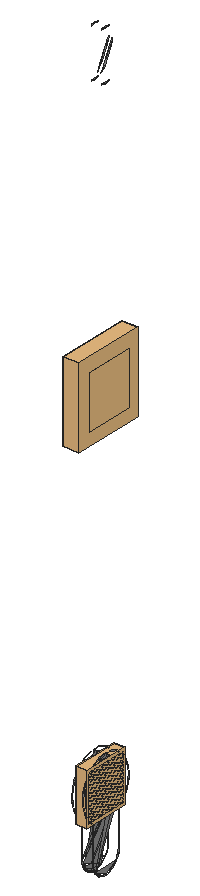
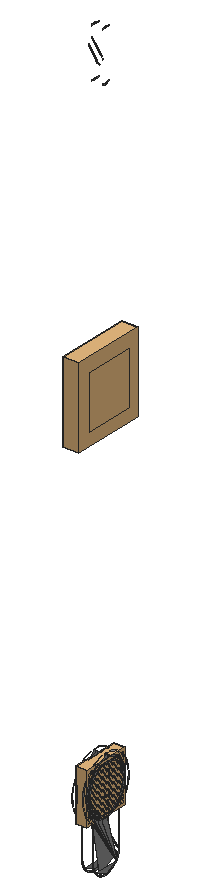
# SketchUp Ruby script. Lengths in inches.
U = 1.inch
M = Sketchup.active_model
def pt(a) = Geom::Point3d.new(a.map { |v| v * U })
def face(e, loops, mat)
  f = e.add_face(loops[0].map { |a| pt(a) })
  loops[1..].each { |l| e.add_face(l.map { |a| pt(a) }).erase! }
  f.material = f.back_material = mat if mat
  f
end
# faces: each face lists its corners as indices into pts; further lists are holes
def faces(e, pts, list, mat = nil) = list.each { |f| face(e, (f[0].is_a?(Array) ? f : [f]).map { |l| l.map { |i| pts[i] } }, mat) }
# xy, xz, yz: faces in a plane at the given z, y or x. An outline is a flat list of corners, or four numbers for a rectangle; further outlines are holes
def ring(l) = l.size == 4 ? [[l[0], l[1]], [l[2], l[1]], [l[2], l[3]], [l[0], l[3]]] : l.each_slice(2).to_a
def flat(e, list, mat, &to3) = list.each { |f| face(e, (f[0].is_a?(Array) ? f : [f]).map { |l| ring(l).map { |u, v| to3.(u, v) } }, mat) }
def xy(e, z, list, mat = nil) = flat(e, list, mat) { |x, y| [x, y, z] }
def xz(e, y, list, mat = nil) = flat(e, list, mat) { |x, z| [x, y, z] }
def yz(e, x, list, mat = nil) = flat(e, list, mat) { |y, z| [x, y, z] }
def lines(e, pts, list) = list.each { |a, b| e.add_line(pt(pts[a]), pt(pts[b])) }
# prism: a flat outline (further loops are holes) pulled along v
def prism(e, loops, v, mat = nil)
  f = face(e, loops, mat); d = Geom::Vector3d.new(v.map { |x| x * U })
  f.pushpull(f.normal.samedirection?(d) ? d.length : -d.length)
end
def box(e, o, s, mat = nil) = prism(e, [[o, [o[0] + s[0], o[1], o[2]], [o[0] + s[0], o[1] + s[1], o[2]], [o[0], o[1] + s[1], o[2]]]], [0, 0, s[2]], mat)
def at(x, y, z, deg = 0) = Geom::Transformation.translation(pt([x, y, z])) * Geom::Transformation.rotation(ORIGIN, Z_AXIS, deg.degrees)
def axes(o, x, y, z) = Geom::Transformation.new([*x, 0, *y, 0, *z, 0, *pt(o).to_a, 1])
def part(name) = M.definitions.add(name)
# library, detail: a bought-in or finely detailed component or shape, given as its bounding box
def library(name, o, s) = part(name).tap { |d| box(d.entities, o, s) }
def detail(e, o, s) = box(e.add_group.entities, o, s)
def put(e, d, t, mat = nil) = e.add_instance(d, t).tap { |i| i.material = mat if mat }
def group(e, t, mat = nil) = e.add_group.tap { |g| g.transformation = t; g.material = mat if mat }.entities
root = M.entities
M.materials.add("Material \#1").color = [140, 140, 140]
c1 = library("3DGeom~1_Defintion",[-60.87,347.29,-704.08],[121.74,121.75,1000])
c2 = library("3DGeom~13_Defintion",[-84.91,-744.98,-830.03],[169.82,169.83,1000])
c3 = library("3DGeom~14_Defintion",[-102.17,352.37,-727.27],[204.35,204.35,1000])
c4 = part("3DGeom~10_Defintion")
yz(c4.entities,-68.96,[[-797.08,-844.83,-797.08,-827.59,-922.41,-827.59],[-922.41,-844.83,-797.08,-844.83,-922.41,-827.59]],"Material \#1")
yz(c4.entities,68.97,[[-922.41,-844.83,-797.08,-827.59,-797.08,-844.83],[-922.41,-844.83,-922.41,-827.59,-797.08,-827.59],[-797.08,137.93,-922.41,155.17,-797.08,155.17],[-922.41,137.93,-922.41,155.17,-797.08,137.93]],"Material \#1")
p = [[-15.8,-989.55,-844.83],[-15.8,-989.55,-827.59],[0,-991.38,-827.59],[0,-991.38,-844.83],[15.8,-989.55,-827.59],[15.8,-989.55,-844.83],
  [-30.32,-984.36,-844.83],[-30.32,-984.36,-827.59],[30.31,-984.36,-827.59],[30.31,-984.36,-844.83],[-43.12,-976.21,-844.83],[-43.12,-976.21,-827.59],
  [43.12,-976.21,-827.59],[43.12,-976.21,-844.83],[-53.81,-965.53,-844.83],[-53.81,-965.53,-827.59],[53.8,-965.53,-827.59],[53.8,-965.53,-844.83],
  [-61.95,-952.73,-844.83],[-61.95,-952.73,-827.59],[53.8,-965.53,-827.59],[61.95,-952.73,-827.59],[61.95,-952.73,-844.83],[-67.15,-938.21,-844.83],
  [-67.15,-938.21,-827.59],[67.14,-938.21,-827.59],[67.14,-938.21,-844.83],[-68.96,-922.41,-844.83],[-68.96,-922.41,-827.59],[67.14,-938.21,-827.59],
  [68.97,-922.41,-827.59],[68.97,-922.41,-844.83],[-69.1,-794.86,-844.83],[-69.1,-794.86,-827.59],[-68.96,-797.08,-827.59],[-68.96,-797.08,-844.83],
  [68.97,-797.08,-844.83],[68.97,-797.08,-827.59],[69.11,-794.71,-827.59],[69.11,-794.71,-844.83],[-69.48,-792.73,-844.83],[-69.48,-792.73,-827.59],
  [69.53,-792.51,-827.59],[69.53,-792.51,-844.83],[-70.14,-790.6875,-844.83],[-70.14,-790.6875,-827.59],[70.24,-790.48,-827.59],[70.24,-790.48,-844.83],
  [-71.08,-788.73,-844.83],[-71.08,-788.73,-827.59],[71.22,-788.57,-827.59],[71.22,-788.57,-844.83],[-72.32,-786.86,-844.83],[-72.32,-786.86,-827.59],
  [72.47,-786.78,-827.59],[72.47,-786.78,-844.83],[-73.8,-785.17,-844.83],[-73.8,-785.17,-827.59],[74,-785.04,-827.59],[74,-785.04,-844.83],
  [-75.96,-783.21,-844.83],[-75.96,-783.21,-827.59],[74,-785.04,-827.59],[75.76,-783.39,-827.59],[75.76,-783.39,-844.83],[86.625,-772.95,-827.59],
  [86.61,-772.96,-844.83],[-86.89,-773.25,-844.83],[-86.89,-773.25,-827.59],[-75.96,-783.21,-844.83],[-96.66,-761.8,-844.83],[-96.66,-761.8,-827.59],
  [86.625,-772.95,-827.59],[86.63,-772.94,-844.83],[86.61,-772.96,-844.83],[86.625,-772.95,-827.59],[86.62,-772.95,-827.59],[86.62,-772.95,-827.59],
  [96.31,-761.375,-827.59],[96.31,-761.375,-844.83],[86.63,-772.94,-844.83],[86.625,-772.95,-827.59],[86.62,-772.95,-827.59],[-104.96,-749.18,-844.83],
  [-104.96,-749.18,-827.59],[-96.66,-761.8,-827.59],[-96.66,-761.8,-844.83],[96.31,-761.375,-827.59],[104.62,-748.77,-827.59],[104.62,-748.77,-844.83],
  [-111.64,-735.52,-844.83],[-111.64,-735.52,-827.59],[111.39,-735.21,-827.59],[111.39,-735.21,-844.83],[-116.49,-721.23,-844.83],[-116.49,-721.23,-827.59],
  [116.4375,-720.78,-827.59],[116.4375,-720.78,-844.83],[-119.64,-705.62,-844.83],[-119.64,-705.62,-827.59],[119.6,-705.57,-827.59],[119.6,-705.57,-844.83],
  [-120.6875,-689.65,-844.83],[-120.6875,-689.65,-827.59],[120.69,-689.65,-827.59],[120.69,-689.65,-844.83],[-117.5,-662,-844.83],[-117.5,-662,-827.59],
  [117.5,-662,-827.59],[117.5,-662,-844.83],[-108.41,-636.61,-844.83],[-108.41,-636.61,-827.59],[117.5,-662,-844.83],[108.41,-636.61,-827.59],
  [108.41,-636.61,-844.83],[-93.91,-613.95,-844.83],[-93.91,-613.95,-827.59],[-108.41,-636.61,-827.59],[108.41,-636.61,-844.83],[94.16,-614.19,-827.59],
  [94.16,-614.19,-844.83],[94.16,-614.19,-827.59],[75.46,-595.5,-827.59],[75.46,-595.5,-844.83],[-75.46,-595.5,-844.83],[-75.46,-595.5,-827.59],
  [-93.91,-613.95,-827.59],[-93.91,-613.95,-827.59],[-93.91,-613.95,-844.83],[-53.05,-581.24,-844.83],[-53.05,-581.24,-827.59],[-75.46,-595.5,-827.59],
  [-75.46,-595.5,-844.83],[53.05,-581.24,-827.59],[53.05,-581.24,-844.83],[-27.65,-572.16,-844.83],[-27.65,-572.16,-827.59],[-53.05,-581.24,-827.59],
  [-53.05,-581.24,-844.83],[27.66,-572.16,-827.59],[27.66,-572.16,-844.83],[0,-568.97,-844.83],[0,-568.97,-827.59],[-27.65,-572.16,-827.59],
  [-27.65,-572.16,-844.83],[0,-568.97,-844.83],[-15.8,-989.55,155.17],[0,-991.38,155.17],[0,-991.38,137.93],[-15.8,-989.55,137.93],
  [15.8,-989.55,155.17],[15.8,-989.55,137.93],[-30.32,-984.36,155.17],[-30.32,-984.36,137.93],[30.31,-984.36,155.17],[30.31,-984.36,137.93],
  [-43.125,-976.22,155.17],[-43.125,-976.22,137.93],[43.12,-976.22,155.17],[43.12,-976.22,137.93],[-53.81,-965.53,155.17],[-53.81,-965.53,137.93],
  [53.8,-965.53,155.17],[53.8,-965.53,137.93],[-61.96,-952.73,155.17],[-61.95,-952.73,137.93],[61.95,-952.73,155.17],[61.95,-952.73,137.93],
  [53.8,-965.53,137.93],[-67.15,-938.21,155.17],[-67.15,-938.21,137.93],[67.14,-938.21,155.17],[67.14,-938.21,137.93],[-68.96,-922.41,155.17],
  [-68.96,-922.41,137.93],[68.97,-922.41,155.17],[68.97,-922.41,137.93],[67.14,-938.21,137.93],[-68.97,-797.08,155.17],[-68.97,-797.08,137.93],
  [-69.1,-794.86,155.17],[-69.1,-794.86,137.93],[68.97,-797.08,155.17],[69.11,-794.71,155.17],[69.11,-794.71,137.93],[68.97,-797.08,137.93],
  [-69.48,-792.73,155.17],[-69.48,-792.73,137.93],[69.53,-792.51,155.17],[69.53,-792.51,137.93],[-70.14,-790.6875,155.17],[-70.14,-790.6875,137.93],
  [70.24,-790.48,155.17],[70.24,-790.48,137.93],[-71.08,-788.73,155.17],[-71.08,-788.73,137.93],[71.22,-788.57,155.17],[71.22,-788.57,137.93],
  [-72.32,-786.86,155.17],[-72.32,-786.86,137.93],[72.47,-786.78,155.17],[72.47,-786.78,137.93],[-73.8,-785.17,155.17],[-73.8,-785.17,137.93],
  [74,-785.04,155.17],[74,-785.04,137.93],[-75.96,-783.21,155.17],[-75.96,-783.21,137.93],[75.76,-783.39,155.17],[75.76,-783.39,137.93],
  [74,-785.04,137.93],[86.61,-772.96,155.17],[86.625,-772.95,137.93],[-86.88,-773.25,155.17],[-75.96,-783.21,155.17],[-86.88,-773.25,137.93],
  [-96.66,-761.8,155.17],[-96.66,-761.8,137.93],[86.63,-772.94,155.17],[86.625,-772.95,137.93],[86.61,-772.96,155.17],[86.62,-772.95,137.93],
  [86.625,-772.95,137.93],[96.31,-761.375,155.17],[96.31,-761.375,137.93],[86.62,-772.95,137.93],[86.63,-772.94,155.17],[86.62,-772.95,137.93],
  [86.625,-772.95,137.93],[-104.96,-749.18,155.17],[-96.66,-761.8,155.17],[-96.66,-761.8,137.93],[-104.96,-749.18,137.93],[104.62,-748.77,155.17],
  [104.62,-748.77,137.93],[96.31,-761.375,137.93],[-111.64,-735.52,155.17],[-111.64,-735.52,137.93],[111.39,-735.21,155.17],[111.39,-735.21,137.93],
  [-116.49,-721.23,155.17],[-116.49,-721.23,137.93],[116.4375,-720.78,155.17],[116.4375,-720.78,137.93],[-119.64,-705.62,155.17],[-119.64,-705.62,137.93],
  [119.6,-705.57,155.17],[119.6,-705.57,137.93],[-120.6875,-689.65,155.17],[-120.6875,-689.65,137.93],[120.69,-689.65,155.17],[120.69,-689.65,137.93],
  [-117.5,-662,155.17],[-117.5,-662,137.93],[117.5,-662,155.17],[117.5,-662,137.93],[-108.41,-636.61,155.17],[-108.41,-636.61,137.93],
  [117.5,-662,155.17],[108.41,-636.61,155.17],[108.41,-636.61,137.93],[-93.91,-613.95,155.17],[-108.41,-636.61,137.93],[-93.91,-613.95,137.93],
  [108.41,-636.61,155.17],[94.16,-614.19,155.17],[94.16,-614.19,137.93],[75.46,-595.5,155.17],[75.46,-595.5,137.93],[94.16,-614.19,137.93],
  [-75.46,-595.5,155.17],[-93.91,-613.95,155.17],[-93.91,-613.95,137.93],[-75.46,-595.5,137.93],[-53.05,-581.24,155.17],[-75.46,-595.5,155.17],
  [-75.46,-595.5,137.93],[-53.05,-581.24,137.93],[53.05,-581.24,155.17],[53.05,-581.24,137.93],[-27.65,-572.16,155.17],[-53.05,-581.24,155.17],
  [-53.05,-581.24,137.93],[-27.65,-572.16,137.93],[27.65,-572.16,155.17],[27.65,-572.16,137.93],[0,-568.97,155.17],[-27.65,-572.16,155.17],
  [-27.65,-572.16,137.93],[0,-568.97,137.93],[0,-568.97,155.17]]
faces(c4.entities,p,[[0,1,2],[2,3,0],[3,2,4],[4,5,3],[6,7,1],[1,0,6],[5,4,8],[8,9,5],
  [10,11,7],[7,6,10],[9,8,12],[12,13,9],[14,15,11],[11,10,14],[13,12,16],[16,17,13],
  [18,19,15],[15,14,18],[17,20,21],[21,22,17],[23,24,19],[19,18,23],[22,21,25],[25,26,22],
  [27,28,24],[24,23,27],[26,29,30],[30,31,26],[32,33,34],[34,35,32],[36,37,38],[38,39,36],
  [40,41,33],[33,32,40],[39,38,42],[42,43,39],[44,45,41],[41,40,44],[43,42,46],[46,47,43],
  [48,49,45],[45,44,48],[47,46,50],[50,51,47],[52,53,49],[49,48,52],[51,50,54],[54,55,51],
  [56,57,53],[53,52,56],[55,54,58],[58,59,55],[60,61,57],[57,56,60],[59,62,63],[63,64,59],
  [64,63,65],[65,66,64],[67,68,61],[61,69,67],[70,71,68],[68,67,70],[72,73,66],[74,75,76],
  [73,77,78],[78,79,73],[80,81,82],[83,84,85],[85,86,83],[79,87,88],[88,89,79],[90,91,84],
  [84,83,90],[89,88,92],[92,93,89],[94,95,91],[91,90,94],[93,92,96],[96,97,93],[98,99,95],
  [95,94,98],[97,96,100],[100,101,97],[102,103,99],[99,98,102],[101,100,104],[104,105,101],[106,107,103],
  [103,102,106],[105,104,108],[108,109,105],[110,111,107],[107,106,110],[112,108,113],[113,114,112],[115,116,117],
  [117,110,115],[118,113,119],[119,120,118],[120,121,122],[122,123,120],[124,125,126],[127,128,124],[129,130,131],
  [131,132,129],[123,122,133],[133,134,123],[135,136,137],[137,138,135],[134,133,139],[139,140,134],[141,142,143],
  [143,144,141],[140,139,142],[142,145,140],[146,147,148],[148,149,146],[147,150,151],[151,148,147],[152,146,149],
  [149,153,152],[150,154,155],[155,151,150],[156,152,153],[153,157,156],[154,158,159],[159,155,154],[160,156,157],
  [157,161,160],[158,162,163],[163,159,158],[164,160,161],[161,165,164],[162,166,167],[167,168,162],[169,164,165],
  [165,170,169],[166,171,172],[172,167,166],[173,169,170],[170,174,173],[171,175,176],[176,177,171],[178,173,174],
  [174,179,178],[180,178,179],[179,181,180],[182,183,184],[184,185,182],[186,180,181],[181,187,186],[183,188,189],
  [189,184,183],[190,186,187],[187,191,190],[188,192,193],[193,189,188],[194,190,191],[191,195,194],[192,196,197],
  [197,193,192],[198,194,195],[195,199,198],[196,200,201],[201,197,196],[202,198,199],[199,203,202],[200,204,205],
  [205,201,200],[206,202,203],[203,207,206],[204,208,209],[209,210,204],[208,211,212],[212,209,208],[213,214,207],
  [207,215,213],[216,213,215],[215,217,216],[211,218,219],[220,221,222],[218,223,224],[224,225,218],[226,227,228],
  [229,230,231],[231,232,229],[223,233,234],[234,235,223],[236,229,232],[232,237,236],[233,238,239],[239,234,233],
  [240,236,237],[237,241,240],[238,242,243],[243,239,238],[244,240,241],[241,245,244],[242,246,247],[247,243,242],
  [248,244,245],[245,249,248],[246,250,251],[251,247,246],[252,248,249],[249,253,252],[250,254,255],[255,251,250],
  [256,252,253],[253,257,256],[258,259,260],[260,255,258],[261,256,262],[262,263,261],[264,265,266],[266,260,264],
  [265,267,268],[268,269,265],[270,271,272],[272,273,270],[274,275,276],[276,277,274],[267,278,279],[279,268,267],
  [280,281,282],[282,283,280],[278,284,285],[285,279,278],[286,287,288],[288,289,286],[284,290,289],[289,285,284]],"Material \#1")
c5 = library("3DGeom~12_Defintion",[-95.68,-755.75,-830.03],[191.36,191.37,1000])
xy(root,47.142,[[362.563,201.771,362.563,201.811,362.582,201.771],[362.582,201.771,362.563,201.811,362.582,201.811],[362.669,201.771,362.669,201.811,362.688,201.811],[362.669,201.771,362.688,201.811,362.688,201.771]],"Material \#1")
xy(root,47.537,[[362.563,201.765,362.582,201.765,362.582,201.83],[362.563,201.765,362.582,201.83,362.563,201.83],[362.669,201.765,362.688,201.765,362.669,201.83],[362.688,201.765,362.688,201.83,362.669,201.83]],"Material \#1")
xz(root,201.765,[[362.563,47.389,362.582,47.389,362.582,47.453],[362.669,47.389,362.688,47.389,362.669,47.453]],"Material \#1")
xz(root,201.771,[[362.563,47.251,362.582,47.251,362.582,47.285],[362.563,47.251,362.582,47.285,362.563,47.285],[362.669,47.251,362.688,47.251,362.669,47.285],[362.688,47.251,362.688,47.285,362.669,47.285]],"Material \#1")
xz(root,201.824,[[362.582,47.214,362.563,47.251,362.582,47.251],[362.669,47.214,362.669,47.251,362.688,47.251]],"Material \#1")
xz(root,201.83,[[362.582,47.473,362.563,47.537,362.582,47.537],[362.669,47.473,362.669,47.537,362.688,47.537]],"Material \#1")
yz(root,362.563,[[201.798,47.076,201.738,47.094,201.735,47.085],[201.798,47.076,201.798,47.086,201.738,47.094],[201.798,47.076,201.86,47.085,201.798,47.086],[201.735,47.085,201.681,47.12,201.677,47.111],[201.735,47.085,201.738,47.094,201.681,47.12],
  [201.86,47.085,201.858,47.094,201.798,47.086],[201.86,47.085,201.919,47.111,201.858,47.094],[201.858,47.094,201.919,47.111,201.914,47.12],[201.677,47.111,201.633,47.16,201.627,47.153],[201.677,47.111,201.681,47.12,201.633,47.16],
  [201.919,47.111,201.969,47.153,201.914,47.12],[201.914,47.12,201.969,47.153,201.962,47.16],[201.627,47.153,201.596,47.213,201.588,47.208],[201.627,47.153,201.633,47.16,201.596,47.213],[201.969,47.153,202.007,47.208,201.962,47.16],
  [201.962,47.16,202.007,47.208,201.999,47.213],[201.588,47.208,201.573,47.274,201.564,47.271],[201.588,47.208,201.596,47.213,201.573,47.274],[202.007,47.208,202.031,47.271,201.999,47.213],[201.999,47.213,202.031,47.271,202.023,47.274],
  [201.564,47.271,201.565,47.34,201.556,47.34],[201.564,47.271,201.573,47.274,201.565,47.34],[202.031,47.271,202.04,47.34,202.023,47.274],[202.023,47.274,202.04,47.34,202.031,47.34],[201.556,47.34,201.565,47.34,201.573,47.405],
  [201.556,47.34,201.573,47.405,201.564,47.408],[202.031,47.34,202.031,47.408,202.023,47.405],[202.031,47.34,202.04,47.34,202.031,47.408],[201.573,47.405,201.596,47.466,201.564,47.408],[202.023,47.405,202.007,47.471,201.999,47.466],
  [202.023,47.405,202.031,47.408,202.007,47.471],[201.564,47.408,201.596,47.466,201.588,47.471],[201.596,47.466,201.633,47.519,201.588,47.471],[201.999,47.466,201.969,47.526,201.962,47.519],[201.999,47.466,202.007,47.471,201.969,47.526],
  [201.588,47.471,201.633,47.519,201.627,47.526],[201.633,47.519,201.681,47.559,201.627,47.526],[201.962,47.519,201.919,47.568,201.914,47.559],[201.962,47.519,201.969,47.526,201.919,47.568],[201.627,47.526,201.681,47.559,201.677,47.568],
  [201.681,47.559,201.738,47.585,201.677,47.568],[201.914,47.559,201.86,47.594,201.858,47.585],[201.914,47.559,201.919,47.568,201.86,47.594],[201.677,47.568,201.738,47.585,201.735,47.594],[201.738,47.585,201.798,47.593,201.735,47.594],
  [201.858,47.585,201.798,47.603,201.798,47.593],[201.858,47.585,201.86,47.594,201.798,47.603],[201.798,47.593,201.798,47.603,201.735,47.594]],"Material \#1")
yz(root,362.564,[[201.798,46.486,201.664,46.557,201.722,46.505],[201.798,46.486,201.932,46.557,201.664,46.557],[201.798,46.486,201.722,46.505,201.758,46.491],[201.722,46.505,201.664,46.557,201.69,46.528],[201.664,46.557,201.626,46.674,201.63,46.631],
  [201.664,46.557,201.63,46.631,201.643,46.591],[201.664,46.557,201.86,47.051,201.798,47.044],[201.664,46.557,201.917,47.074,201.86,47.051],[201.664,46.557,201.968,47.109,201.917,47.074],[201.664,46.557,201.97,47.04,201.971,47.047],
  [201.664,46.557,201.971,47.047,201.973,47.054],[201.664,46.557,201.973,47.054,201.976,47.061],[201.664,46.557,202.01,47.155,201.968,47.109],[201.86,47.628,201.798,47.675,201.798,47.635]],"Material \#1")
yz(root,362.566,[[201.798,54.302,201.753,54.321,201.751,54.307],[201.798,54.302,201.798,54.317,201.753,54.321],[201.798,54.302,201.845,54.307,201.798,54.317],[201.845,54.307,201.842,54.321,201.798,54.317],[201.753,54.856,201.798,54.86,201.751,54.87],
  [201.842,54.856,201.798,54.875,201.798,54.86],[201.842,54.856,201.845,54.87,201.798,54.875],[201.798,54.86,201.798,54.875,201.751,54.87]],"Material \#1")
yz(root,362.568,[[201.798,47.044,201.73,47.063,201.727,47.054],[201.798,47.044,201.798,47.054,201.73,47.063],[201.798,47.044,201.868,47.054,201.798,47.054],[201.727,47.054,201.667,47.092,201.662,47.083],[201.727,47.054,201.73,47.063,201.667,47.092],
  [201.798,47.054,201.868,47.054,201.866,47.063],[201.868,47.054,201.934,47.083,201.866,47.063],[201.866,47.063,201.934,47.083,201.929,47.092],[201.662,47.083,201.612,47.137,201.606,47.13],[201.662,47.083,201.667,47.092,201.612,47.137],
  [201.934,47.083,201.99,47.13,201.929,47.092],[201.929,47.092,201.99,47.13,201.983,47.137],[201.606,47.13,201.571,47.197,201.5625,47.192],[201.606,47.13,201.612,47.137,201.571,47.197],[201.99,47.13,202.033,47.192,201.983,47.137],
  [201.983,47.137,202.033,47.192,202.025,47.197],[201.5625,47.192,201.544,47.266,201.536,47.263],[201.5625,47.192,201.571,47.197,201.544,47.266],[202.033,47.192,202.06,47.263,202.025,47.197],[202.025,47.197,202.06,47.263,202.051,47.266],
  [201.536,47.263,201.535,47.34,201.526,47.34],[201.536,47.263,201.544,47.266,201.535,47.34],[202.06,47.263,202.069,47.34,202.051,47.266],[202.051,47.266,202.069,47.34,202.06,47.34],[201.526,47.34,201.535,47.34,201.544,47.414],
  [201.526,47.34,201.544,47.414,201.536,47.416],[202.06,47.34,202.06,47.416,202.051,47.414],[202.06,47.34,202.069,47.34,202.06,47.416],[201.544,47.414,201.571,47.482,201.536,47.416],[202.051,47.414,202.033,47.487,202.025,47.482],
  [202.051,47.414,202.06,47.416,202.033,47.487],[201.536,47.416,201.571,47.482,201.5625,47.487],[201.571,47.482,201.612,47.542,201.5625,47.487],[202.025,47.482,201.99,47.549,201.983,47.542],[202.025,47.482,202.033,47.487,201.99,47.549],
  [201.5625,47.487,201.612,47.542,201.606,47.549],[201.612,47.542,201.667,47.587,201.606,47.549],[201.983,47.542,201.934,47.596,201.929,47.587],[201.983,47.542,201.99,47.549,201.934,47.596],[201.606,47.549,201.667,47.587,201.662,47.596],
  [201.667,47.587,201.73,47.616,201.662,47.596],[201.929,47.587,201.868,47.625,201.866,47.616],[201.929,47.587,201.934,47.596,201.868,47.625],[201.662,47.596,201.73,47.616,201.727,47.625],[201.73,47.616,201.798,47.625,201.727,47.625],
  [201.866,47.616,201.798,47.635,201.798,47.625],[201.866,47.616,201.868,47.625,201.798,47.635],[201.727,47.625,201.798,47.625,201.798,47.635]],"Material \#1")
yz(root,362.582,[[201.771,47.142,201.811,47.142,201.784,47.172],[201.811,47.142,201.824,47.172,201.784,47.172],[201.784,47.172,201.824,47.172,201.777,47.182],[201.824,47.172,201.831,47.182,201.777,47.182],[201.777,47.182,201.831,47.182,201.777,47.204],
  [201.831,47.182,201.831,47.204,201.777,47.204],[201.777,47.204,201.831,47.204,201.784,47.214],[201.831,47.204,201.824,47.214,201.784,47.214],[201.784,47.214,201.824,47.214,201.771,47.251],[201.824,47.214,201.824,47.251,201.771,47.251],
  [201.771,47.251,201.824,47.251,201.771,47.285],[201.824,47.251,201.824,47.285,201.771,47.285],[201.771,47.285,201.824,47.285,201.761,47.313],[201.824,47.285,201.834,47.313,201.761,47.313],[201.761,47.313,201.834,47.313,201.761,47.341],
  [201.834,47.313,201.834,47.341,201.761,47.341],[201.761,47.341,201.834,47.341,201.771,47.369],[201.834,47.341,201.824,47.369,201.771,47.369],[201.771,47.369,201.824,47.369,201.765,47.389],[201.824,47.369,201.83,47.389,201.765,47.389],
  [201.765,47.389,201.83,47.389,201.765,47.453],[201.83,47.389,201.83,47.453,201.765,47.453],[201.765,47.453,201.83,47.453,201.773,47.458],[201.83,47.453,201.822,47.458,201.773,47.458],[201.773,47.458,201.822,47.458,201.773,47.468],
  [201.822,47.458,201.822,47.468,201.773,47.468],[201.773,47.468,201.822,47.468,201.765,47.473],[201.822,47.468,201.83,47.473,201.765,47.473],[201.765,47.473,201.83,47.473,201.765,47.537],[201.83,47.473,201.83,47.537,201.765,47.537]],"Material \#1")
yz(root,362.585,[[201.798,46.486,201.722,46.505,201.873,46.505],[201.873,46.505,201.63,46.631,201.97,47.032],[201.626,46.674,201.86,47.051,201.917,47.074],[201.736,47.628,201.798,47.675,201.798,47.635]],"Material \#1")
yz(root,362.667,[[201.798,46.486,201.873,46.505,201.722,46.505],[201.626,46.674,201.917,47.074,201.86,47.051],[201.736,47.628,201.798,47.635,201.798,47.675],[201.86,47.628,201.798,47.675,201.798,47.635]],"Material \#1")
yz(root,362.669,[[201.771,47.142,201.784,47.172,201.811,47.142],[201.811,47.142,201.784,47.172,201.824,47.172],[201.784,47.172,201.777,47.182,201.824,47.172],[201.824,47.172,201.777,47.182,201.831,47.182],[201.777,47.182,201.777,47.204,201.831,47.182],
  [201.831,47.182,201.777,47.204,201.831,47.204],[201.777,47.204,201.784,47.214,201.831,47.204],[201.831,47.204,201.784,47.214,201.824,47.214],[201.784,47.214,201.771,47.251,201.824,47.214],[201.824,47.214,201.771,47.251,201.824,47.251],
  [201.771,47.251,201.771,47.285,201.824,47.251],[201.824,47.251,201.771,47.285,201.824,47.285],[201.771,47.285,201.761,47.313,201.824,47.285],[201.824,47.285,201.761,47.313,201.834,47.313],[201.761,47.313,201.761,47.341,201.834,47.313],
  [201.834,47.313,201.761,47.341,201.834,47.341],[201.761,47.341,201.771,47.369,201.834,47.341],[201.834,47.341,201.771,47.369,201.824,47.369],[201.771,47.369,201.765,47.389,201.824,47.369],[201.824,47.369,201.765,47.389,201.83,47.389],
  [201.765,47.389,201.765,47.453,201.83,47.389],[201.83,47.389,201.765,47.453,201.83,47.453],[201.765,47.453,201.773,47.458,201.83,47.453],[201.83,47.453,201.773,47.458,201.822,47.458],[201.773,47.458,201.773,47.468,201.822,47.458],
  [201.822,47.458,201.773,47.468,201.822,47.468],[201.773,47.468,201.765,47.473,201.822,47.468],[201.822,47.468,201.765,47.473,201.83,47.473],[201.765,47.473,201.765,47.537,201.83,47.473],[201.83,47.473,201.765,47.537,201.83,47.537]],"Material \#1")
yz(root,362.683,[[201.798,47.044,201.727,47.054,201.73,47.063],[201.798,47.044,201.73,47.063,201.798,47.054],[201.798,47.044,201.798,47.054,201.868,47.054],[201.727,47.054,201.662,47.083,201.667,47.092],[201.727,47.054,201.667,47.092,201.73,47.063],
  [201.798,47.054,201.866,47.063,201.868,47.054],[201.868,47.054,201.866,47.063,201.934,47.083],[201.866,47.063,201.929,47.092,201.934,47.083],[201.662,47.083,201.606,47.13,201.612,47.137],[201.662,47.083,201.612,47.137,201.667,47.092],
  [201.934,47.083,201.929,47.092,201.99,47.13],[201.929,47.092,201.983,47.137,201.99,47.13],[201.606,47.13,201.5625,47.192,201.571,47.197],[201.606,47.13,201.571,47.197,201.612,47.137],[201.99,47.13,201.983,47.137,202.033,47.192],
  [201.983,47.137,202.025,47.197,202.033,47.192],[201.5625,47.192,201.536,47.263,201.544,47.266],[201.5625,47.192,201.544,47.266,201.571,47.197],[202.033,47.192,202.025,47.197,202.06,47.263],[202.025,47.197,202.051,47.266,202.06,47.263],
  [201.536,47.263,201.526,47.34,201.535,47.34],[201.536,47.263,201.535,47.34,201.544,47.266],[202.06,47.263,202.051,47.266,202.069,47.34],[202.051,47.266,202.06,47.34,202.069,47.34],[201.526,47.34,201.536,47.416,201.544,47.414],
  [201.526,47.34,201.544,47.414,201.535,47.34],[202.06,47.34,202.051,47.414,202.06,47.416],[202.06,47.34,202.06,47.416,202.069,47.34],[201.544,47.414,201.536,47.416,201.571,47.482],[202.051,47.414,202.025,47.482,202.033,47.487],
  [202.051,47.414,202.033,47.487,202.06,47.416],[201.536,47.416,201.5625,47.487,201.571,47.482],[201.571,47.482,201.5625,47.487,201.612,47.542],[202.025,47.482,201.983,47.542,201.99,47.549],[202.025,47.482,201.99,47.549,202.033,47.487],
  [201.5625,47.487,201.606,47.549,201.612,47.542],[201.612,47.542,201.606,47.549,201.667,47.587],[201.983,47.542,201.929,47.587,201.934,47.596],[201.983,47.542,201.934,47.596,201.99,47.549],[201.606,47.549,201.662,47.596,201.667,47.587],
  [201.667,47.587,201.662,47.596,201.73,47.616],[201.929,47.587,201.866,47.616,201.868,47.625],[201.929,47.587,201.868,47.625,201.934,47.596],[201.662,47.596,201.727,47.625,201.73,47.616],[201.73,47.616,201.727,47.625,201.798,47.625],
  [201.866,47.616,201.798,47.625,201.798,47.635],[201.866,47.616,201.798,47.635,201.868,47.625],[201.727,47.625,201.798,47.635,201.798,47.625]],"Material \#1")
yz(root,362.685,[[201.798,54.302,201.751,54.307,201.753,54.321],[201.798,54.302,201.753,54.321,201.798,54.317],[201.798,54.302,201.798,54.317,201.845,54.307],[201.845,54.307,201.798,54.317,201.842,54.321],[201.753,54.856,201.751,54.87,201.798,54.86],
  [201.842,54.856,201.798,54.86,201.798,54.875],[201.842,54.856,201.798,54.875,201.845,54.87],[201.798,54.86,201.751,54.87,201.798,54.875]],"Material \#1")
yz(root,362.6875,[[201.798,46.486,201.664,46.557,201.932,46.557],[201.664,46.557,201.798,47.044,201.86,47.051],[201.664,46.557,201.86,47.051,201.917,47.074],[201.736,47.628,201.798,47.675,201.798,47.635],[201.86,47.628,201.798,47.635,201.798,47.675]],"Material \#1")
p = [[362.563,201.771,47.142],[362.582,201.771,47.142],[362.582,201.784,47.172],[362.582,201.784,47.172],[362.563,201.781,47.177],[362.563,201.771,47.142],
  [362.563,201.827,47.177],[362.582,201.824,47.172],[362.582,201.811,47.142],[362.563,201.811,47.142],[362.563,201.827,47.177],[362.669,201.784,47.172],
  [362.669,201.771,47.142],[362.688,201.771,47.142],[362.688,201.771,47.142],[362.688,201.781,47.177],[362.669,201.784,47.172],[362.688,201.827,47.177],
  [362.688,201.811,47.142],[362.669,201.811,47.142],[362.669,201.824,47.172],[362.688,201.827,47.177],[362.582,201.771,47.251],[362.563,201.771,47.251],
  [362.563,201.781,47.209],[362.563,201.781,47.209],[362.582,201.784,47.214],[362.582,201.771,47.251],[362.563,201.781,47.177],[362.582,201.777,47.182],
  [362.582,201.777,47.204],[362.563,201.781,47.209],[362.563,201.781,47.177],[362.582,201.784,47.172],[362.582,201.777,47.182],[362.563,201.781,47.209],
  [362.582,201.777,47.204],[362.582,201.784,47.214],[362.582,201.824,47.214],[362.563,201.827,47.209],[362.563,201.824,47.251],[362.563,201.827,47.177],
  [362.582,201.831,47.182],[362.582,201.824,47.172],[362.563,201.827,47.209],[362.582,201.824,47.214],[362.582,201.831,47.204],[362.563,201.827,47.209],
  [362.582,201.831,47.204],[362.582,201.831,47.182],[362.563,201.827,47.177],[362.688,201.781,47.209],[362.688,201.771,47.251],[362.669,201.771,47.251],
  [362.669,201.771,47.251],[362.669,201.784,47.214],[362.688,201.781,47.209],[362.688,201.781,47.177],[362.688,201.781,47.209],[362.669,201.777,47.204],
  [362.669,201.777,47.182],[362.688,201.781,47.177],[362.669,201.777,47.182],[362.669,201.784,47.172],[362.688,201.781,47.209],[362.669,201.784,47.214],
  [362.669,201.777,47.204],[362.688,201.824,47.251],[362.688,201.827,47.209],[362.669,201.824,47.214],[362.688,201.827,47.177],[362.669,201.824,47.172],
  [362.669,201.831,47.182],[362.688,201.827,47.209],[362.669,201.831,47.204],[362.669,201.824,47.214],[362.688,201.827,47.209],[362.688,201.827,47.177],
  [362.669,201.831,47.182],[362.669,201.831,47.204],[362.563,201.771,47.285],[362.582,201.771,47.285],[362.582,201.761,47.313],[362.582,201.771,47.369],
  [362.563,201.771,47.369],[362.563,201.761,47.341],[362.582,201.824,47.251],[362.563,201.824,47.251],[362.563,201.829,47.299],[362.563,201.829,47.299],
  [362.582,201.824,47.285],[362.582,201.824,47.251],[362.563,201.827,47.379],[362.582,201.824,47.369],[362.582,201.834,47.341],[362.582,201.824,47.285],
  [362.563,201.829,47.299],[362.563,201.834,47.327],[362.582,201.834,47.341],[362.563,201.829,47.355],[362.563,201.827,47.379],[362.563,201.834,47.327],
  [362.582,201.834,47.313],[362.582,201.824,47.285],[362.582,201.834,47.313],[362.563,201.834,47.327],[362.563,201.829,47.355],[362.563,201.829,47.355],
  [362.582,201.834,47.341],[362.582,201.834,47.313],[362.688,201.771,47.285],[362.688,201.761,47.313],[362.669,201.761,47.313],[362.669,201.771,47.285],
  [362.688,201.761,47.341],[362.688,201.771,47.369],[362.669,201.771,47.369],[362.669,201.824,47.251],[362.669,201.824,47.285],[362.688,201.829,47.299],
  [362.688,201.829,47.299],[362.688,201.824,47.251],[362.669,201.824,47.251],[362.669,201.834,47.341],[362.669,201.824,47.369],[362.688,201.827,47.379],
  [362.688,201.834,47.327],[362.688,201.829,47.299],[362.669,201.824,47.285],[362.688,201.827,47.379],[362.688,201.829,47.355],[362.669,201.834,47.341],
  [362.669,201.824,47.285],[362.669,201.834,47.313],[362.688,201.834,47.327],[362.688,201.829,47.355],[362.688,201.834,47.327],[362.669,201.834,47.313],
  [362.669,201.834,47.313],[362.669,201.834,47.341],[362.688,201.829,47.355],[362.582,201.765,47.453],[362.563,201.768,47.465],[362.563,201.765,47.389],
  [362.582,201.765,47.389],[362.563,201.765,47.389],[362.563,201.771,47.369],[362.563,201.771,47.369],[362.582,201.771,47.369],[362.582,201.765,47.389],
  [362.582,201.824,47.369],[362.563,201.827,47.379],[362.563,201.83,47.393],[362.563,201.83,47.393],[362.582,201.83,47.389],[362.582,201.824,47.369],
  [362.582,201.83,47.389],[362.563,201.83,47.393],[362.563,201.827,47.458],[362.563,201.827,47.458],[362.582,201.83,47.453],[362.582,201.83,47.389],
  [362.688,201.765,47.389],[362.688,201.768,47.465],[362.669,201.765,47.453],[362.688,201.771,47.369],[362.688,201.765,47.389],[362.669,201.765,47.389],
  [362.669,201.765,47.389],[362.669,201.771,47.369],[362.688,201.771,47.369],[362.688,201.83,47.393],[362.688,201.827,47.379],[362.669,201.824,47.369],
  [362.669,201.824,47.369],[362.669,201.83,47.389],[362.688,201.83,47.393],[362.688,201.827,47.458],[362.688,201.83,47.393],[362.669,201.83,47.389],
  [362.669,201.83,47.389],[362.669,201.83,47.453],[362.688,201.827,47.458],[362.582,201.765,47.537],[362.563,201.765,47.537],[362.563,201.768,47.465],
  [362.563,201.768,47.465],[362.582,201.765,47.473],[362.582,201.765,47.537],[362.563,201.768,47.465],[362.582,201.765,47.453],[362.582,201.773,47.458],
  [362.563,201.827,47.458],[362.582,201.822,47.468],[362.582,201.822,47.458],[362.563,201.827,47.458],[362.582,201.83,47.473],[362.563,201.827,47.458],
  [362.582,201.83,47.453],[362.563,201.768,47.465],[362.582,201.773,47.468],[362.582,201.765,47.473],[362.563,201.768,47.465],[362.582,201.83,47.473],
  [362.563,201.827,47.458],[362.563,201.83,47.537],[362.688,201.768,47.465],[362.688,201.765,47.537],[362.669,201.765,47.537],[362.669,201.765,47.537],
  [362.669,201.765,47.473],[362.688,201.768,47.465],[362.688,201.768,47.465],[362.669,201.773,47.458],[362.669,201.765,47.453],[362.688,201.827,47.458],
  [362.669,201.822,47.458],[362.669,201.822,47.468],[362.688,201.827,47.458],[362.669,201.83,47.473],[362.688,201.827,47.458],[362.669,201.83,47.453],
  [362.688,201.768,47.465],[362.669,201.765,47.473],[362.669,201.773,47.468],[362.688,201.768,47.465],[362.688,201.83,47.537],[362.688,201.827,47.458],
  [362.669,201.83,47.473],[362.566,201.767,54.464],[362.568,201.767,54.464],[362.568,201.75,54.431],[362.566,201.75,54.431],[362.568,201.721,54.444],
  [362.566,201.721,54.444],[362.568,201.696,54.465],[362.566,201.696,54.465],[362.685,201.767,54.464],[362.685,201.75,54.431],[362.683,201.75,54.431],
  [362.684,201.767,54.464],[362.685,201.721,54.444],[362.683,201.721,54.444],[362.685,201.696,54.465],[362.683,201.696,54.465],[362.568,201.714,54.497],
  [362.566,201.714,54.497],[362.567,201.73,54.526],[362.566,201.73,54.526],[362.567,201.813,54.684],[362.566,201.813,54.684],[362.685,201.714,54.497],
  [362.684,201.714,54.497],[362.685,201.73,54.526],[362.684,201.73,54.526],[362.685,201.813,54.684],[362.684,201.813,54.684],[362.566,201.866,54.651],
  [362.567,201.866,54.651],[362.567,201.782,54.493],[362.566,201.782,54.493],[362.685,201.866,54.651],[362.685,201.782,54.493],[362.684,201.782,54.493],
  [362.684,201.866,54.651],[362.568,201.828,54.713],[362.566,201.828,54.713],[362.568,201.846,54.746],[362.566,201.846,54.746],[362.568,201.874,54.733],
  [362.566,201.874,54.733],[362.685,201.828,54.713],[362.684,201.828,54.713],[362.685,201.846,54.746],[362.683,201.846,54.746],[362.685,201.874,54.733],
  [362.683,201.874,54.733],[362.568,201.899,54.713],[362.566,201.899,54.713],[362.568,201.882,54.68],[362.566,201.882,54.68],[362.685,201.899,54.713],
  [362.683,201.899,54.713],[362.685,201.882,54.68],[362.684,201.882,54.68]]
faces(root,p,[[0,1,2],[3,4,5],[6,7,8],[8,9,10],[11,12,13],[14,15,16],[17,18,19],[19,20,21],
  [22,23,24],[25,26,27],[28,29,30],[30,31,28],[32,33,34],[35,36,37],[38,39,40],[41,42,43],
  [44,45,46],[47,48,49],[49,50,47],[51,52,53],[54,55,56],[57,58,59],[59,60,57],[61,62,63],
  [64,65,66],[67,68,69],[70,71,72],[73,74,75],[76,77,78],[78,79,76],[80,81,82],[83,84,85],
  [86,87,88],[89,90,91],[92,93,94],[95,96,97],[98,99,100],[101,102,103],[104,105,106],[107,108,109],
  [110,111,112],[112,113,110],[114,115,116],[117,118,119],[120,121,122],[123,124,125],[126,127,128],[129,130,131],
  [132,133,134],[135,136,137],[138,139,140],[141,142,143],[144,145,146],[147,148,149],[150,151,152],[153,154,155],
  [156,157,158],[159,160,161],[162,163,164],[165,166,167],[168,169,170],[171,172,173],[174,175,176],[177,178,179],
  [180,181,182],[183,184,185],[186,187,188],[189,190,191],[192,193,194],[195,196,193],[197,194,198],[199,200,201],
  [202,191,200],[203,204,205],[206,207,208],[209,210,211],[212,213,214],[215,216,217],[218,217,219],[220,221,216],
  [222,223,224],[225,224,213],[226,227,228],[229,230,231],[231,232,229],[232,231,233],[233,234,232],[234,233,235],
  [235,236,234],[237,238,239],[239,240,237],[238,241,242],[242,239,238],[241,243,244],[244,242,241],[236,235,245],
  [245,246,236],[246,245,247],[247,248,246],[248,247,249],[249,250,248],[243,251,252],[252,244,243],[251,253,254],
  [254,252,251],[253,255,256],[256,254,253],[257,258,259],[259,260,257],[260,259,230],[230,229,260],[261,262,263],
  [263,264,261],[262,237,240],[240,263,262],[250,249,265],[265,266,250],[266,265,267],[267,268,266],[268,267,269],
  [269,270,268],[255,271,272],[272,256,255],[271,273,274],[274,272,271],[273,275,276],[276,274,273],[270,269,277],
  [277,278,270],[278,277,279],[279,280,278],[280,279,258],[258,257,280],[275,281,282],[282,276,275],[281,283,284],
  [284,282,281],[283,261,264],[264,284,283]],"Material \#1")
put(root,c1,axes([362.67,201.8,49.3125],[0,-0.00443,0],[0,0,0.00483],[0.0002,0,0]),"Material \#1")
put(root,c2,axes([362.67,201.8,49.3125],[0,-0.00274,0],[0,0,0.00299],[0.00012,0,0]),"Material \#1")
put(root,c3,axes([362.67,201.8,49.3125],[0,-0.00398,0],[0,0,0.00434],[0.00018,0,0]),"Material \#1")
put(root,c4,axes([362.67,201.8,49.3125],[0,-0.00262,0],[0,0,0.00286],[0.00012,0,0]),"Material \#1")
put(root,c5,axes([362.67,201.8,49.3125],[0,-0.00274,0],[0,0,0.00299],[0.00012,0,0]),"Material \#1")
